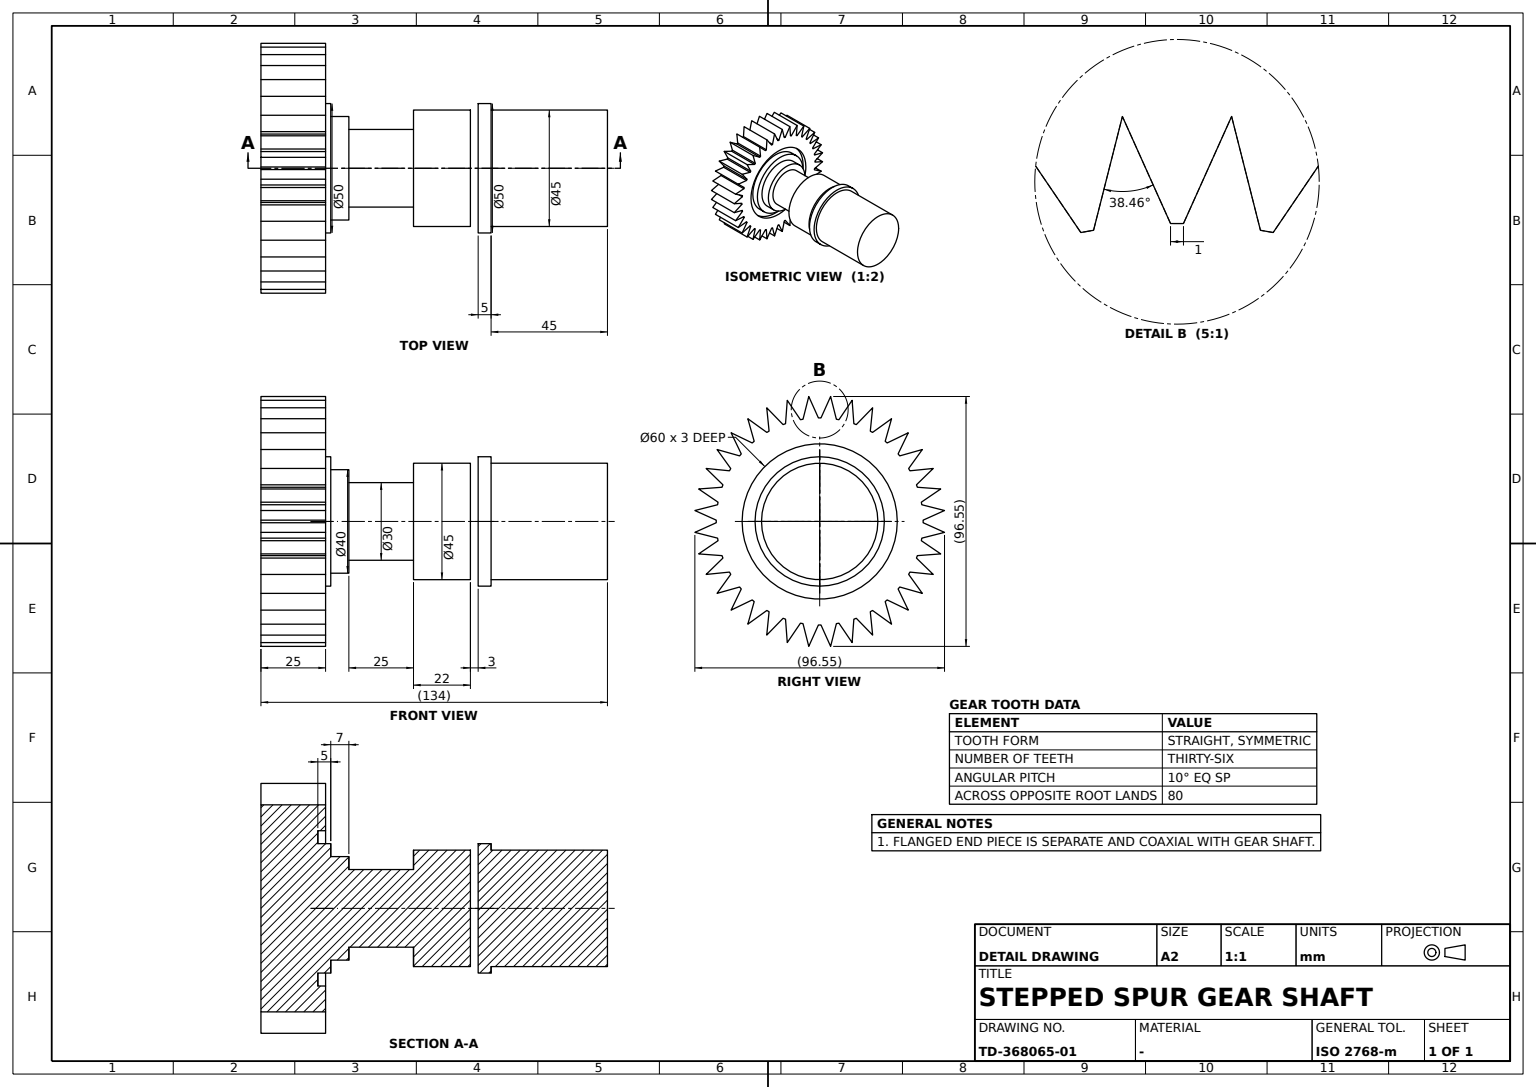
solid
v1 (89,-22.5,0)
v2 (134,-22.5,0)
e1 v1 v2 LINE
v3 (89,22.5,0)
e2 v1 v3 CIRCLE(AX(P(89,0,0),D(1,0,0),D(0,1,0)),22.5)
v4 (134,22.5,0)
e3 v3 v4 LINE
e4 v2 v4 CIRCLE(AX(P(134,0,0),D(1,0,0),D(0,1,0)),22.5)
face CYL(AX(P(71.5,0,0),D(-1,0,0),D(0,1,0)),22.5) [-e1 e2 e3 -e4]
e5 v4 v2 CIRCLE(AX(P(134,0,0),D(1,0,0),D(0,1,0)),22.5)
face PLANE(AX(P(134,0,0),D(1,0,0),D(0,1,0))) [e4 e5]
v5 (84,25,0)
v6 (84,-25,0)
e6 v5 v6 CIRCLE(AX(P(84,0,0),D(1,0,0),D(0,1,0)),25)
v7 (89,-25,0)
e7 v6 v7 LINE
v8 (89,25,0)
e8 v8 v7 CIRCLE(AX(P(89,0,0),D(1,0,0),D(0,1,0)),25)
e9 v5 v8 LINE
face CYL(AX(P(24.5,0,0),D(-1,0,0),D(0,1,0)),25) [e6 e7 -e8 -e9]
e10 v7 v8 CIRCLE(AX(P(89,0,0),D(1,0,0),D(0,1,0)),25)
e11 v3 v1 CIRCLE(AX(P(89,0,0),D(1,0,0),D(0,1,0)),22.5)
face PLANE(AX(P(89,0,0),D(1,0,0),D(0,1,0))) [e10 e8] [-e2 -e11]
face CYL(AX(P(71.5,0,0),D(-1,0,0),D(0,1,0)),22.5) [-e5 -e3 e11 e1]
e12 v6 v5 CIRCLE(AX(P(84,0,0),D(1,0,0),D(0,1,0)),25)
face PLANE(AX(P(84,0,0),D(1,0,0),D(0,1,0))) rev [-e12 -e6]
face CYL(AX(P(24.5,0,0),D(-1,0,0),D(0,1,0)),25) [e9 -e10 -e7 e12]
solid
v9 (0,-39.695086,27.794799)
v10 (25,-39.695086,27.794799)
e13 v9 v10 LINE
v11 (25,-30.963172,25.328482)
e14 v10 v11 LINE
v12 (0,-30.963172,25.328482)
e15 v11 v12 LINE
e16 v9 v12 LINE
face PLANE(AX(P(25,-30.963172,25.328482),D(0,-0.271814264,-0.962349732),D(0,-0.962349732,0.271814264))) rev [e13 e14 e15 -e16]
v13 (25,34.391016,-20.433013)
v14 (0,34.391016,-20.433013)
e17 v13 v14 LINE
v15 (25,39.695086,-27.794799)
e18 v13 v15 LINE
v16 (0,39.695086,-27.794799)
e19 v16 v15 LINE
e20 v14 v16 LINE
face PLANE(AX(P(25,34.391016,-20.433013),D(0,0.811346988,0.584564851),D(0,0.584564851,-0.811346988))) [-e17 e18 -e19 -e20]
v17 (25,-27.794799,-39.695086)
v18 (25,-25.328482,-30.963172)
e21 v17 v18 LINE
v19 (0,-25.328482,-30.963172)
e22 v18 v19 LINE
v20 (0,-27.794799,-39.695086)
e23 v20 v19 LINE
e24 v20 v17 LINE
face PLANE(AX(P(25,-25.328482,-30.963172),D(0,0.962349732,-0.271814264),D(0,-0.271814264,-0.962349732))) rev [e21 e22 -e23 e24]
v21 (0,-20.433013,-34.391016)
e25 v21 v20 LINE
v22 (25,-20.433013,-34.391016)
e26 v22 v21 LINE
e27 v22 v17 LINE
face PLANE(AX(P(25,-20.433013,-34.391016),D(0,0.584564851,-0.811346988),D(0,-0.811346988,-0.584564851))) [-e24 -e25 -e26 e27]
v23 (25,-30.320384,-26.094527)
v24 (0,-30.320384,-26.094527)
e28 v23 v24 LINE
v25 (25,-30.963172,-25.328482)
e29 v23 v25 LINE
v26 (0,-30.963172,-25.328482)
e30 v25 v26 LINE
e31 v24 v26 LINE
face PLANE(AX(P(25,-30.963172,-25.328482),D(0,0.766044443,0.64278761),D(0,0.64278761,-0.766044443))) rev [-e28 e29 e30 -e31]
v27 (27,20,0)
v28 (27,-20,0)
e32 v27 v28 CIRCLE(AX(P(27,0,0),D(1,0,0),D(0,1,0)),20)
e33 v28 v27 CIRCLE(AX(P(27,0,0),D(1,0,0),D(0,1,0)),20)
v29 (27,-25,0)
v30 (27,25,0)
e34 v29 v30 CIRCLE(AX(P(27,0,0),D(1,0,0),D(0,1,0)),25)
e35 v30 v29 CIRCLE(AX(P(27,0,0),D(1,0,0),D(0,1,0)),25)
face PLANE(AX(P(27,0,0),D(1,0,0),D(0,1,0))) [-e32 -e33] [e34 e35]
v31 (0,4.223459,-48.274352)
v32 (25,4.223459,-48.274352)
e36 v31 v32 LINE
v33 (25,0.5,-40)
e37 v32 v33 LINE
v34 (0,0.5,-40)
e38 v33 v34 LINE
e39 v31 v34 LINE
face PLANE(AX(P(25,0.5,-40),D(0,0.911921505,0.410364677),D(0,0.410364677,-0.911921505))) rev [e36 e37 e38 -e39]
v35 (25,-13.210959,37.758715)
v36 (0,-13.210959,37.758715)
e40 v35 v36 LINE
v37 (25,-12.542048,46.807561)
e41 v35 v37 LINE
v38 (0,-12.542048,46.807561)
e42 v38 v37 LINE
e43 v36 v38 LINE
face PLANE(AX(P(25,-13.210959,37.758715),D(0,-0.997278895,0.073721135),D(0,0.073721135,0.997278895))) [-e40 e41 -e42 -e43]
v39 (0,37.758715,-13.210959)
v40 (0,37.416695,-14.150652)
e44 v39 v40 LINE
v41 (25,37.758715,-13.210959)
e45 v41 v39 LINE
v42 (25,37.416695,-14.150652)
e46 v41 v42 LINE
e47 v42 v40 LINE
face PLANE(AX(P(25,37.416695,-14.150652),D(0,-0.939692621,0.342020143),D(0,0.342020143,0.939692621))) rev [-e44 -e45 e46 e47]
v43 (25,20.479554,43.918545)
v44 (25,19.566987,34.891016)
e48 v43 v44 LINE
v45 (0,19.566987,34.891016)
e49 v44 v45 LINE
v46 (0,20.479554,43.918545)
e50 v46 v45 LINE
e51 v46 v43 LINE
face PLANE(AX(P(25,19.566987,34.891016),D(0,-0.994929528,0.100574517),D(0,0.100574517,0.994929528))) rev [e48 e49 -e50 e51]
v47 (25,37.416695,14.150652)
v48 (0,37.416695,14.150652)
e52 v47 v48 LINE
v49 (25,37.758715,13.210959)
e53 v47 v49 LINE
v50 (0,37.758715,13.210959)
e54 v49 v50 LINE
e55 v48 v50 LINE
face PLANE(AX(P(25,37.758715,13.210959),D(0,-0.939692621,-0.342020143),D(0,-0.342020143,0.939692621))) rev [-e52 e53 e54 -e55]
v51 (0,-19.566987,-34.891016)
e56 v51 v21 LINE
v52 (25,-19.566987,-34.891016)
e57 v52 v51 LINE
e58 v52 v22 LINE
face PLANE(AX(P(25,-20.433013,-34.391016),D(0,0.5,0.866025404),D(0,0.866025404,-0.5))) rev [e26 -e56 -e57 e58]
v53 (25,34.891016,19.566987)
v54 (0,34.891016,19.566987)
e59 v53 v54 LINE
v55 (0,34.391016,20.433013)
e60 v55 v54 LINE
v56 (25,34.391016,20.433013)
e61 v56 v55 LINE
e62 v56 v53 LINE
face PLANE(AX(P(25,34.891016,19.566987),D(0,-0.866025404,-0.5),D(0,-0.5,0.866025404))) rev [e59 -e60 -e61 e62]
v57 (0,27.794799,-39.695086)
v58 (25,27.794799,-39.695086)
e63 v57 v58 LINE
v59 (25,20.433013,-34.391016)
e64 v58 v59 LINE
v60 (0,20.433013,-34.391016)
e65 v59 v60 LINE
e66 v57 v60 LINE
face PLANE(AX(P(25,20.433013,-34.391016),D(0,0.584564851,0.811346988),D(0,0.811346988,-0.584564851))) rev [e63 e64 e65 -e66]
v61 (25,-37.416695,14.150652)
v62 (25,-43.918545,20.479554)
e67 v61 v62 LINE
v63 (0,-43.918545,20.479554)
e68 v63 v62 LINE
v64 (0,-37.416695,14.150652)
e69 v64 v63 LINE
e70 v61 v64 LINE
face PLANE(AX(P(25,-37.416695,14.150652),D(0,-0.697512183,-0.716572923),D(0,-0.716572923,0.697512183))) [e67 -e68 -e69 -e70]
v65 (25,-37.758715,13.210959)
e71 v65 v61 LINE
v66 (0,-37.758715,13.210959)
e72 v66 v64 LINE
e73 v65 v66 LINE
face PLANE(AX(P(25,-37.416695,14.150652),D(0,0.939692621,-0.342020143),D(0,-0.342020143,-0.939692621))) rev [e71 e70 -e72 -e73]
v67 (0,-0.5,-40)
e74 v34 v67 LINE
v68 (25,-0.5,-40)
e75 v33 v68 LINE
e76 v68 v67 LINE
face PLANE(AX(P(25,-0.5,-40),D(0,0,1),D(0,1,0))) rev [-e74 -e38 e75 e76]
v69 (25,12.542048,-46.807561)
v70 (25,7.438331,-39.305486)
e77 v69 v70 LINE
v71 (0,7.438331,-39.305486)
e78 v70 v71 LINE
v72 (0,12.542048,-46.807561)
e79 v72 v71 LINE
e80 v72 v69 LINE
face PLANE(AX(P(25,7.438331,-39.305486),D(0,0.82680829,0.562483823),D(0,0.562483823,-0.82680829))) rev [e77 e78 -e79 e80]
v73 (25,40,0.5)
v74 (25,40,-0.5)
e81 v73 v74 LINE
v75 (0,40,-0.5)
e82 v74 v75 LINE
v76 (0,40,0.5)
e83 v76 v75 LINE
e84 v73 v76 LINE
face PLANE(AX(P(25,40,-0.5),D(0,-1,0),D(0,0,1))) rev [e81 e82 -e83 -e84]
v77 (25,30.963172,-25.328482)
e85 v15 v77 LINE
v78 (0,30.963172,-25.328482)
e86 v77 v78 LINE
e87 v16 v78 LINE
face PLANE(AX(P(25,30.963172,-25.328482),D(0,0.271814264,0.962349732),D(0,0.962349732,-0.271814264))) rev [e85 e86 -e87 e19]
v79 (0,-34.265513,-34.265513)
v80 (25,-34.265513,-34.265513)
e88 v79 v80 LINE
v81 (0,-26.094527,-30.320384)
e89 v81 v79 LINE
v82 (25,-26.094527,-30.320384)
e90 v82 v81 LINE
e91 v82 v80 LINE
face PLANE(AX(P(25,-26.094527,-30.320384),D(0,0.434795072,-0.900529425),D(0,-0.900529425,-0.434795072))) [-e88 -e89 -e90 e91]
v83 (0,-46.807561,-12.542048)
v84 (0,-39.305486,-7.438331)
e92 v83 v84 LINE
v85 (25,-46.807561,-12.542048)
e93 v83 v85 LINE
v86 (25,-39.305486,-7.438331)
e94 v85 v86 LINE
e95 v86 v84 LINE
face PLANE(AX(P(25,-39.305486,-7.438331),D(0,0.562483823,-0.82680829),D(0,-0.82680829,-0.562483823))) rev [-e92 e93 e94 e95]
v87 (25,-25.328482,30.963172)
v88 (0,-25.328482,30.963172)
e96 v87 v88 LINE
v89 (25,-27.794799,39.695086)
e97 v87 v89 LINE
v90 (0,-27.794799,39.695086)
e98 v90 v89 LINE
e99 v88 v90 LINE
face PLANE(AX(P(25,-25.328482,30.963172),D(0,-0.962349732,-0.271814264),D(0,-0.271814264,0.962349732))) [-e96 e97 -e98 -e99]
v91 (22,-25,0)
v92 (22,25,0)
e100 v91 v92 CIRCLE(AX(P(22,0,0),D(1,0,0),D(0,1,0)),25)
e101 v92 v91 CIRCLE(AX(P(22,0,0),D(1,0,0),D(0,1,0)),25)
v93 (22,-30,0)
v94 (22,30,0)
e102 v93 v94 CIRCLE(AX(P(22,0,0),D(1,0,0),D(0,1,0)),30)
e103 v94 v93 CIRCLE(AX(P(22,0,0),D(1,0,0),D(0,1,0)),30)
face PLANE(AX(P(22,0,0),D(1,0,0),D(0,1,0))) [-e100 -e101] [e102 e103]
v95 (25,-40,-0.5)
v96 (25,-40,0.5)
e104 v95 v96 LINE
v97 (0,-40,0.5)
e105 v96 v97 LINE
v98 (0,-40,-0.5)
e106 v98 v97 LINE
e107 v95 v98 LINE
face PLANE(AX(P(25,-40,0.5),D(0,1,0),D(0,0,-1))) rev [e104 e105 -e106 -e107]
v99 (0,39.695086,27.794799)
e108 v99 v55 LINE
v100 (25,39.695086,27.794799)
e109 v99 v100 LINE
e110 v100 v56 LINE
face PLANE(AX(P(25,34.391016,20.433013),D(0,-0.811346988,0.584564851),D(0,0.584564851,0.811346988))) rev [e61 -e108 e109 e110]
v101 (25,12.542048,46.807561)
v102 (25,13.210959,37.758715)
e111 v101 v102 LINE
v103 (0,13.210959,37.758715)
e112 v102 v103 LINE
v104 (0,12.542048,46.807561)
e113 v104 v103 LINE
e114 v104 v101 LINE
face PLANE(AX(P(25,13.210959,37.758715),D(0,-0.997278895,-0.073721135),D(0,-0.073721135,0.997278895))) rev [e111 e112 -e113 e114]
v105 (0,19.566987,-34.891016)
v106 (0,20.479554,-43.918545)
e115 v105 v106 LINE
v107 (25,19.566987,-34.891016)
e116 v107 v105 LINE
v108 (25,20.479554,-43.918545)
e117 v107 v108 LINE
e118 v106 v108 LINE
face PLANE(AX(P(25,19.566987,-34.891016),D(0,0.994929528,0.100574517),D(0,0.100574517,-0.994929528))) [-e115 -e116 e117 -e118]
v109 (25,43.918545,-20.479554)
e119 v42 v109 LINE
v110 (0,43.918545,-20.479554)
e120 v110 v109 LINE
e121 v40 v110 LINE
face PLANE(AX(P(25,37.416695,-14.150652),D(0,0.697512183,0.716572923),D(0,0.716572923,-0.697512183))) [e119 -e120 -e121 -e47]
v111 (0,-19.566987,34.891016)
v112 (0,-20.479554,43.918545)
e122 v111 v112 LINE
v113 (25,-19.566987,34.891016)
e123 v113 v111 LINE
v114 (25,-20.479554,43.918545)
e124 v113 v114 LINE
e125 v112 v114 LINE
face PLANE(AX(P(25,-19.566987,34.891016),D(0,-0.994929528,-0.100574517),D(0,-0.100574517,0.994929528))) [-e122 -e123 e124 -e125]
v115 (25,30.320384,-26.094527)
e126 v77 v115 LINE
v116 (0,30.320384,-26.094527)
e127 v115 v116 LINE
e128 v78 v116 LINE
face PLANE(AX(P(25,30.320384,-26.094527),D(0,-0.766044443,0.64278761),D(0,0.64278761,0.766044443))) rev [e126 e127 -e128 -e86]
v117 (0,-20.433013,34.391016)
e129 v117 v111 LINE
v118 (25,-20.433013,34.391016)
e130 v118 v117 LINE
e131 v118 v113 LINE
face PLANE(AX(P(25,-19.566987,34.891016),D(0,0.5,-0.866025404),D(0,-0.866025404,-0.5))) rev [e123 -e129 -e130 e131]
e132 v90 v117 LINE
e133 v89 v118 LINE
face PLANE(AX(P(25,-20.433013,34.391016),D(0,-0.584564851,-0.811346988),D(0,-0.811346988,0.584564851))) rev [-e132 e98 e133 e130]
e134 v91 v29 LINE
e135 v92 v30 LINE
face CYL(AX(P(24.5,0,0),D(-1,0,0),D(0,1,0)),25) [e101 e134 -e35 -e135]
v119 (25,14.150652,-37.416695)
e136 v108 v119 LINE
v120 (0,14.150652,-37.416695)
e137 v119 v120 LINE
e138 v106 v120 LINE
face PLANE(AX(P(25,14.150652,-37.416695),D(0,0.716572923,0.697512183),D(0,0.697512183,-0.716572923))) rev [e136 e137 -e138 e118]
v121 (25,-48.274352,4.223459)
e139 v96 v121 LINE
v122 (0,-48.274352,4.223459)
e140 v122 v121 LINE
e141 v97 v122 LINE
face PLANE(AX(P(25,-40,0.5),D(0,-0.410364677,-0.911921505),D(0,-0.911921505,0.410364677))) [-e105 e139 -e140 -e141]
v123 (25,6.453523,39.479134)
v124 (0,6.453523,39.479134)
e142 v123 v124 LINE
v125 (25,7.438331,39.305486)
e143 v123 v125 LINE
v126 (0,7.438331,39.305486)
e144 v125 v126 LINE
e145 v124 v126 LINE
face PLANE(AX(P(25,7.438331,39.305486),D(0,-0.173648178,-0.984807753),D(0,-0.984807753,0.173648178))) rev [-e142 e143 e144 -e145]
v127 (25,-34.891016,19.566987)
e146 v62 v127 LINE
v128 (0,-34.891016,19.566987)
e147 v127 v128 LINE
e148 v63 v128 LINE
face PLANE(AX(P(25,-34.891016,19.566987),D(0,-0.100574517,-0.994929528),D(0,-0.994929528,0.100574517))) rev [e68 e146 e147 -e148]
v129 (25,20.433013,34.391016)
e149 v44 v129 LINE
v130 (0,20.433013,34.391016)
e150 v129 v130 LINE
e151 v45 v130 LINE
face PLANE(AX(P(25,20.433013,34.391016),D(0,-0.5,-0.866025404),D(0,-0.866025404,0.5))) rev [e149 e150 -e151 -e49]
v131 (25,-14.150652,37.416695)
e152 v131 v35 LINE
v132 (0,-14.150652,37.416695)
e153 v132 v36 LINE
e154 v131 v132 LINE
face PLANE(AX(P(25,-13.210959,37.758715),D(0,0.342020143,-0.939692621),D(0,-0.939692621,-0.342020143))) rev [e152 e40 -e153 -e154]
v133 (25,-7.438331,39.305486)
v134 (25,-6.453523,39.479134)
e155 v133 v134 LINE
v135 (0,-6.453523,39.479134)
e156 v134 v135 LINE
v136 (0,-7.438331,39.305486)
e157 v136 v135 LINE
e158 v133 v136 LINE
face PLANE(AX(P(25,-6.453523,39.479134),D(0,0.173648178,-0.984807753),D(0,-0.984807753,-0.173648178))) rev [e155 e156 -e157 -e158]
v137 (25,-34.391016,20.433013)
e159 v137 v10 LINE
v138 (0,-34.391016,20.433013)
e160 v138 v9 LINE
e161 v137 v138 LINE
face PLANE(AX(P(25,-34.391016,20.433013),D(0,-0.811346988,-0.584564851),D(0,-0.584564851,0.811346988))) [e159 -e13 -e160 -e161]
v139 (25,6.453523,-39.479134)
e162 v139 v32 LINE
v140 (0,6.453523,-39.479134)
e163 v140 v31 LINE
e164 v139 v140 LINE
face PLANE(AX(P(25,6.453523,-39.479134),D(0,0.969326447,-0.245776808),D(0,-0.245776808,-0.969326447))) [e162 -e36 -e163 -e164]
v141 (34,20,0)
v142 (34,-20,0)
e165 v141 v142 CIRCLE(AX(P(34,0,0),D(1,0,0),D(0,1,0)),20)
e166 v142 v141 CIRCLE(AX(P(34,0,0),D(1,0,0),D(0,1,0)),20)
v143 (34,15,0)
v144 (34,-15,0)
e167 v143 v144 CIRCLE(AX(P(34,0,0),D(1,0,0),D(0,1,0)),15)
e168 v144 v143 CIRCLE(AX(P(34,0,0),D(1,0,0),D(0,1,0)),15)
face PLANE(AX(P(34,0,0),D(1,0,0),D(0,1,0))) [e165 e166] [-e167 -e168]
v145 (0,39.305486,7.438331)
v146 (0,39.479134,6.453523)
e169 v145 v146 LINE
v147 (25,39.305486,7.438331)
e170 v147 v145 LINE
v148 (25,39.479134,6.453523)
e171 v147 v148 LINE
e172 v148 v146 LINE
face PLANE(AX(P(25,39.479134,6.453523),D(0,-0.984807753,-0.173648178),D(0,-0.173648178,0.984807753))) rev [-e169 -e170 e171 e172]
v149 (0,-46.807561,12.542048)
v150 (25,-46.807561,12.542048)
e173 v149 v150 LINE
e174 v150 v65 LINE
e175 v149 v66 LINE
face PLANE(AX(P(25,-37.758715,13.210959),D(0,0.073721135,-0.997278895),D(0,-0.997278895,-0.073721135))) rev [e173 e174 e73 -e175]
v151 (0,25.328482,-30.963172)
e176 v151 v57 LINE
v152 (25,25.328482,-30.963172)
e177 v152 v151 LINE
e178 v152 v58 LINE
face PLANE(AX(P(25,25.328482,-30.963172),D(0,0.962349732,0.271814264),D(0,0.271814264,-0.962349732))) [-e63 -e176 -e177 e178]
v153 (25,34.265513,-34.265513)
e179 v115 v153 LINE
v154 (0,34.265513,-34.265513)
e180 v154 v153 LINE
e181 v116 v154 LINE
face PLANE(AX(P(25,30.320384,-26.094527),D(0,0.900529425,0.434795072),D(0,0.434795072,-0.900529425))) [e179 -e180 -e181 -e127]
v155 (25,-37.416695,-14.150652)
v156 (25,-37.758715,-13.210959)
e182 v155 v156 LINE
v157 (0,-37.758715,-13.210959)
e183 v156 v157 LINE
v158 (0,-37.416695,-14.150652)
e184 v158 v157 LINE
e185 v155 v158 LINE
face PLANE(AX(P(25,-37.758715,-13.210959),D(0,0.939692621,0.342020143),D(0,0.342020143,-0.939692621))) rev [e182 e183 -e184 -e185]
v159 (25,-34.391016,-20.433013)
v160 (25,-34.891016,-19.566987)
e186 v159 v160 LINE
v161 (0,-34.891016,-19.566987)
e187 v160 v161 LINE
v162 (0,-34.391016,-20.433013)
e188 v162 v161 LINE
e189 v159 v162 LINE
face PLANE(AX(P(25,-34.891016,-19.566987),D(0,0.866025404,0.5),D(0,0.5,-0.866025404))) rev [e186 e187 -e188 -e189]
v163 (25,39.305486,-7.438331)
v164 (25,46.807561,-12.542048)
e190 v163 v164 LINE
v165 (0,46.807561,-12.542048)
e191 v165 v164 LINE
v166 (0,39.305486,-7.438331)
e192 v166 v165 LINE
e193 v163 v166 LINE
face PLANE(AX(P(25,39.305486,-7.438331),D(0,0.562483823,0.82680829),D(0,0.82680829,-0.562483823))) [e190 -e191 -e192 -e193]
v167 (0,-6.453523,-39.479134)
v168 (0,-7.438331,-39.305486)
e194 v167 v168 LINE
v169 (25,-6.453523,-39.479134)
e195 v169 v167 LINE
v170 (25,-7.438331,-39.305486)
e196 v169 v170 LINE
e197 v170 v168 LINE
face PLANE(AX(P(25,-7.438331,-39.305486),D(0,0.173648178,0.984807753),D(0,0.984807753,-0.173648178))) rev [-e194 -e195 e196 e197]
v171 (25,13.210959,-37.758715)
e198 v119 v171 LINE
v172 (0,13.210959,-37.758715)
e199 v171 v172 LINE
e200 v120 v172 LINE
face PLANE(AX(P(25,13.210959,-37.758715),D(0,-0.342020143,0.939692621),D(0,0.939692621,0.342020143))) rev [-e137 e198 e199 -e200]
v173 (25,48.274352,-4.223459)
e201 v74 v173 LINE
v174 (0,48.274352,-4.223459)
e202 v174 v173 LINE
e203 v75 v174 LINE
face PLANE(AX(P(25,40,-0.5),D(0,0.410364677,0.911921505),D(0,0.911921505,-0.410364677))) [-e82 e201 -e202 -e203]
e204 v171 v69 LINE
e205 v172 v72 LINE
face PLANE(AX(P(25,13.210959,-37.758715),D(0,0.997278895,-0.073721135),D(0,-0.073721135,-0.997278895))) [-e199 e204 -e80 -e205]
v175 (25,-39.479134,6.453523)
v176 (0,-39.479134,6.453523)
e206 v175 v176 LINE
v177 (25,-39.305486,7.438331)
e207 v175 v177 LINE
v178 (0,-39.305486,7.438331)
e208 v177 v178 LINE
e209 v176 v178 LINE
face PLANE(AX(P(25,-39.305486,7.438331),D(0,0.984807753,-0.173648178),D(0,-0.173648178,-0.984807753))) rev [-e206 e207 e208 -e209]
v179 (0,48.274352,4.223459)
e210 v179 v76 LINE
v180 (25,48.274352,4.223459)
e211 v179 v180 LINE
e212 v180 v73 LINE
face PLANE(AX(P(25,40,0.5),D(0,-0.410364677,0.911921505),D(0,0.911921505,0.410364677))) rev [e84 -e210 e211 e212]
v181 (25,26.094527,-30.320384)
v182 (0,26.094527,-30.320384)
e213 v181 v182 LINE
e214 v154 v182 LINE
e215 v153 v181 LINE
face PLANE(AX(P(25,26.094527,-30.320384),D(0,0.434795072,0.900529425),D(0,0.900529425,-0.434795072))) rev [e213 -e214 e180 e215]
v183 (25,25.328482,30.963172)
v184 (25,26.094527,30.320384)
e216 v183 v184 LINE
v185 (0,26.094527,30.320384)
e217 v184 v185 LINE
v186 (0,25.328482,30.963172)
e218 v186 v185 LINE
e219 v183 v186 LINE
face PLANE(AX(P(25,26.094527,30.320384),D(0,-0.64278761,-0.766044443),D(0,-0.766044443,0.64278761))) rev [e216 e217 -e218 -e219]
v187 (0,30.963172,25.328482)
e220 v187 v99 LINE
v188 (25,30.963172,25.328482)
e221 v188 v187 LINE
e222 v188 v100 LINE
face PLANE(AX(P(25,30.963172,25.328482),D(0,-0.271814264,0.962349732),D(0,0.962349732,0.271814264))) [-e220 -e221 e222 -e109]
v189 (25,34.891016,-19.566987)
e223 v109 v189 LINE
v190 (0,34.891016,-19.566987)
e224 v189 v190 LINE
e225 v110 v190 LINE
face PLANE(AX(P(25,34.891016,-19.566987),D(0,0.100574517,0.994929528),D(0,0.994929528,-0.100574517))) rev [e223 e224 -e225 e120]
e226 v79 v24 LINE
e227 v80 v23 LINE
face PLANE(AX(P(25,-30.320384,-26.094527),D(0,0.900529425,-0.434795072),D(0,-0.434795072,-0.900529425))) rev [-e226 e88 e227 e28]
v191 (25,-30.320384,26.094527)
v192 (0,-30.320384,26.094527)
e228 v191 v192 LINE
v193 (25,-34.265513,34.265513)
e229 v191 v193 LINE
v194 (0,-34.265513,34.265513)
e230 v194 v193 LINE
e231 v192 v194 LINE
face PLANE(AX(P(25,-30.320384,26.094527),D(0,-0.900529425,-0.434795072),D(0,-0.434795072,0.900529425))) [-e228 e229 -e230 -e231]
e232 v156 v85 LINE
e233 v157 v83 LINE
face PLANE(AX(P(25,-37.758715,-13.210959),D(0,-0.073721135,-0.997278895),D(0,-0.997278895,0.073721135))) [e232 -e93 -e233 -e183]
v195 (25,43.918545,20.479554)
e234 v195 v47 LINE
v196 (0,43.918545,20.479554)
e235 v196 v48 LINE
e236 v196 v195 LINE
face PLANE(AX(P(25,37.416695,14.150652),D(0,-0.697512183,0.716572923),D(0,0.716572923,0.697512183))) rev [e234 e52 -e235 e236]
v197 (0,34.265513,34.265513)
v198 (0,30.320384,26.094527)
e237 v197 v198 LINE
v199 (25,34.265513,34.265513)
e238 v197 v199 LINE
v200 (25,30.320384,26.094527)
e239 v199 v200 LINE
e240 v200 v198 LINE
face PLANE(AX(P(25,30.320384,26.094527),D(0,-0.900529425,0.434795072),D(0,0.434795072,0.900529425))) rev [-e237 e238 e239 e240]
v201 (0,-4.223459,48.274352)
v202 (0,-0.5,40)
e241 v201 v202 LINE
v203 (25,-4.223459,48.274352)
e242 v201 v203 LINE
v204 (25,-0.5,40)
e243 v203 v204 LINE
e244 v204 v202 LINE
face PLANE(AX(P(25,-0.5,40),D(0,-0.911921505,-0.410364677),D(0,-0.410364677,0.911921505))) rev [-e241 e242 e243 e244]
e245 v165 v39 LINE
e246 v164 v41 LINE
face PLANE(AX(P(25,37.758715,-13.210959),D(0,-0.073721135,0.997278895),D(0,0.997278895,0.073721135))) rev [-e245 e191 e246 e45]
e247 v27 v141 LINE
e248 v28 v142 LINE
face CYL(AX(P(30.5,0,0),D(-1,0,0),D(0,1,0)),20) [e247 -e166 -e248 e33]
v205 (0,4.223459,48.274352)
v206 (25,4.223459,48.274352)
e249 v205 v206 LINE
v207 (0,0.5,40)
e250 v207 v205 LINE
v208 (25,0.5,40)
e251 v208 v207 LINE
e252 v208 v206 LINE
face PLANE(AX(P(25,0.5,40),D(0,-0.911921505,0.410364677),D(0,0.410364677,0.911921505))) [-e249 -e250 -e251 e252]
v209 (0,46.807561,12.542048)
v210 (25,46.807561,12.542048)
e253 v209 v210 LINE
e254 v50 v209 LINE
e255 v49 v210 LINE
face PLANE(AX(P(25,37.758715,13.210959),D(0,0.073721135,0.997278895),D(0,0.997278895,-0.073721135))) [-e253 -e254 -e54 e255]
e256 v12 v192 LINE
e257 v11 v191 LINE
face PLANE(AX(P(25,-30.320384,26.094527),D(0,0.766044443,-0.64278761),D(0,-0.64278761,-0.766044443))) rev [-e256 -e15 e257 e228]
e258 v198 v187 LINE
e259 v200 v188 LINE
face PLANE(AX(P(25,30.963172,25.328482),D(0,-0.766044443,-0.64278761),D(0,-0.64278761,0.766044443))) rev [-e258 -e240 e259 e221]
v211 (59,22.5,0)
v212 (81,22.5,0)
e260 v211 v212 LINE
v213 (81,-22.5,0)
e261 v213 v212 CIRCLE(AX(P(81,0,0),D(1,0,0),D(0,1,0)),22.5)
v214 (59,-22.5,0)
e262 v214 v213 LINE
e263 v214 v211 CIRCLE(AX(P(59,0,0),D(1,0,0),D(0,1,0)),22.5)
face CYL(AX(P(71.5,0,0),D(-1,0,0),D(0,1,0)),22.5) [e260 -e261 -e262 e263]
v215 (25,-30,0)
v216 (25,30,0)
e264 v215 v216 CIRCLE(AX(P(25,0,0),D(1,0,0),D(0,1,0)),30)
e265 v216 v94 LINE
e266 v215 v93 LINE
face CYL(AX(P(23.5,0,0),D(-1,0,0),D(0,1,0)),30) rev [e264 e265 -e102 -e266]
e267 v182 v151 LINE
e268 v181 v152 LINE
face PLANE(AX(P(25,25.328482,-30.963172),D(0,-0.64278761,0.766044443),D(0,0.766044443,0.64278761))) rev [e177 -e267 -e213 e268]
e269 v204 v208 LINE
e270 v202 v207 LINE
face PLANE(AX(P(25,0.5,40),D(0,0,-1),D(0,-1,0))) rev [e269 e251 -e270 -e244]
v217 (0,-39.695086,-27.794799)
v218 (25,-39.695086,-27.794799)
e271 v217 v218 LINE
e272 v218 v159 LINE
e273 v217 v162 LINE
face PLANE(AX(P(25,-34.391016,-20.433013),D(0,0.811346988,-0.584564851),D(0,-0.584564851,-0.811346988))) rev [e271 e272 e189 -e273]
e274 v211 v214 CIRCLE(AX(P(59,0,0),D(1,0,0),D(0,1,0)),22.5)
e275 v212 v213 CIRCLE(AX(P(81,0,0),D(1,0,0),D(0,1,0)),22.5)
face CYL(AX(P(71.5,0,0),D(-1,0,0),D(0,1,0)),22.5) [e274 e262 -e275 -e260]
v219 (59,15,0)
e276 v143 v219 LINE
v220 (59,-15,0)
e277 v220 v219 CIRCLE(AX(P(59,0,0),D(1,0,0),D(0,1,0)),15)
e278 v144 v220 LINE
face CYL(AX(P(46.5,0,0),D(-1,0,0),D(0,1,0)),15) [e276 -e277 -e278 e168]
v221 (0,-26.094527,30.320384)
e279 v221 v88 LINE
v222 (25,-26.094527,30.320384)
e280 v222 v221 LINE
e281 v222 v87 LINE
face PLANE(AX(P(25,-25.328482,30.963172),D(0,0.64278761,-0.766044443),D(0,-0.766044443,-0.64278761))) rev [e96 -e279 -e280 e281]
face PLANE(AX(P(81,0,0),D(1,0,0),D(0,1,0))) [e275 e261]
e282 v219 v220 CIRCLE(AX(P(59,0,0),D(1,0,0),D(0,1,0)),15)
face CYL(AX(P(46.5,0,0),D(-1,0,0),D(0,1,0)),15) [-e282 -e276 e167 e278]
e283 v60 v105 LINE
e284 v71 v140 LINE
v223 (0,-4.223459,-48.274352)
e285 v67 v223 LINE
e286 v223 v167 LINE
v224 (0,-12.542048,-46.807561)
e287 v168 v224 LINE
v225 (0,-13.210959,-37.758715)
e288 v224 v225 LINE
v226 (0,-14.150652,-37.416695)
e289 v225 v226 LINE
v227 (0,-20.479554,-43.918545)
e290 v226 v227 LINE
e291 v227 v51 LINE
e292 v19 v81 LINE
e293 v26 v217 LINE
v228 (0,-43.918545,-20.479554)
e294 v161 v228 LINE
e295 v228 v158 LINE
v229 (0,-39.479134,-6.453523)
e296 v84 v229 LINE
v230 (0,-48.274352,-4.223459)
e297 v229 v230 LINE
e298 v230 v98 LINE
e299 v122 v176 LINE
e300 v178 v149 LINE
e301 v128 v138 LINE
e302 v194 v221 LINE
e303 v112 v132 LINE
e304 v38 v136 LINE
e305 v135 v201 LINE
e306 v205 v124 LINE
e307 v126 v104 LINE
v231 (0,14.150652,37.416695)
e308 v103 v231 LINE
e309 v231 v46 LINE
v232 (0,27.794799,39.695086)
e310 v130 v232 LINE
e311 v232 v186 LINE
e312 v185 v197 LINE
e313 v54 v196 LINE
e314 v209 v145 LINE
e315 v146 v179 LINE
v233 (0,39.479134,-6.453523)
e316 v174 v233 LINE
e317 v233 v166 LINE
e318 v190 v14 LINE
face PLANE(AX(P(0,0,0),D(1,0,0),D(0,1,0))) rev [e87 e128 e181 e214 e267 e176 e66 e283 e115 e138 e200 e205 e79 e284 e163 e39 e74 e285 e286 e194 e287 e288 e289 e290 e291 e56 e25 e23 e292 e89 e226 e31 e293 e273 e188 e294 e295 e184 e233 e92 e296 e297 e298 e106 e141 e299 e209 e300 e175 e72 e69 e148 e301 e160 e16 e256 e231 e302 e279 e99 e132 e129 e122 e303 e153 e43 e304 e157 e305 e241 e270 e250 e306 e145 e307 e113 e308 e309 e50 e151 e310 e311 e218 e312 e237 e258 e220 e108 e60 e313 e235 e55 e254 e314 e169 e315 e210 e83 e203 e316 e317 e192 e245 e44 e121 e225 e318 e20]
e319 v127 v137 LINE
face PLANE(AX(P(25,-34.391016,20.433013),D(0,0.866025404,-0.5),D(0,-0.5,-0.866025404))) rev [-e301 -e147 e319 e161]
v234 (25,39.479134,-6.453523)
e320 v234 v233 LINE
e321 v234 v163 LINE
face PLANE(AX(P(25,39.305486,-7.438331),D(0,-0.984807753,0.173648178),D(0,0.173648178,0.984807753))) rev [e193 -e317 -e320 e321]
e322 v125 v101 LINE
face PLANE(AX(P(25,7.438331,39.305486),D(0,-0.82680829,0.562483823),D(0,0.562483823,0.82680829))) [-e307 -e144 e322 -e114]
v235 (25,-12.542048,-46.807561)
v236 (25,-13.210959,-37.758715)
e323 v235 v236 LINE
e324 v236 v225 LINE
e325 v224 v235 LINE
face PLANE(AX(P(25,-13.210959,-37.758715),D(0,0.997278895,0.073721135),D(0,0.073721135,-0.997278895))) rev [e323 e324 -e288 e325]
e326 v210 v147 LINE
face PLANE(AX(P(25,39.305486,7.438331),D(0,-0.562483823,0.82680829),D(0,0.82680829,0.562483823))) rev [-e314 e253 e326 e170]
v237 (25,14.150652,37.416695)
e327 v237 v231 LINE
e328 v102 v237 LINE
face PLANE(AX(P(25,14.150652,37.416695),D(0,-0.342020143,-0.939692621),D(0,-0.939692621,0.342020143))) rev [e327 -e308 -e112 e328]
e329 v25 v218 LINE
face PLANE(AX(P(25,-30.963172,-25.328482),D(0,0.271814264,-0.962349732),D(0,-0.962349732,-0.271814264))) [-e293 -e30 e329 -e271]
e330 v59 v107 LINE
face PLANE(AX(P(25,19.566987,-34.891016),D(0,-0.5,0.866025404),D(0,0.866025404,0.5))) rev [-e65 e330 e116 -e283]
v238 (25,-43.918545,-20.479554)
e331 v228 v238 LINE
e332 v160 v238 LINE
face PLANE(AX(P(25,-34.891016,-19.566987),D(0,0.100574517,-0.994929528),D(0,-0.994929528,-0.100574517))) [-e331 -e294 -e187 e332]
e333 v134 v203 LINE
face PLANE(AX(P(25,-6.453523,39.479134),D(0,-0.969326447,0.245776808),D(0,0.245776808,0.969326447))) [e333 -e242 -e305 -e156]
e334 v173 v234 LINE
face PLANE(AX(P(25,39.479134,-6.453523),D(0,-0.245776808,0.969326447),D(0,0.969326447,0.245776808))) rev [e202 e334 e320 -e316]
v239 (25,-39.479134,-6.453523)
e335 v239 v229 LINE
v240 (25,-48.274352,-4.223459)
e336 v239 v240 LINE
e337 v230 v240 LINE
face PLANE(AX(P(25,-39.479134,-6.453523),D(0,-0.245776808,-0.969326447),D(0,-0.969326447,0.245776808))) [-e297 -e335 e336 -e337]
v241 (25,-14.150652,-37.416695)
e338 v236 v241 LINE
e339 v241 v226 LINE
face PLANE(AX(P(25,-14.150652,-37.416695),D(0,0.342020143,0.939692621),D(0,0.939692621,-0.342020143))) rev [-e289 -e324 e338 e339]
e340 v86 v239 LINE
face PLANE(AX(P(25,-39.479134,-6.453523),D(0,0.984807753,0.173648178),D(0,0.173648178,-0.984807753))) rev [e335 -e296 -e95 e340]
e341 v177 v150 LINE
face PLANE(AX(P(25,-39.305486,7.438331),D(0,-0.562483823,-0.82680829),D(0,-0.82680829,0.562483823))) [e341 -e173 -e300 -e208]
e342 v189 v13 LINE
face PLANE(AX(P(25,34.391016,-20.433013),D(0,-0.866025404,0.5),D(0,0.5,0.866025404))) rev [-e318 -e224 e342 e17]
e343 v70 v139 LINE
face PLANE(AX(P(25,6.453523,-39.479134),D(0,-0.173648178,0.984807753),D(0,0.984807753,0.173648178))) rev [e164 -e284 -e78 e343]
face PLANE(AX(P(59,0,0),D(1,0,0),D(0,1,0))) rev [e282 e277] [-e263 -e274]
e344 v148 v180 LINE
e345 v53 v195 LINE
e346 v184 v199 LINE
v242 (25,27.794799,39.695086)
e347 v242 v183 LINE
e348 v129 v242 LINE
e349 v237 v43 LINE
e350 v206 v123 LINE
e351 v37 v133 LINE
e352 v114 v131 LINE
e353 v193 v222 LINE
e354 v121 v175 LINE
e355 v240 v95 LINE
e356 v238 v155 LINE
e357 v18 v82 LINE
v243 (25,-20.479554,-43.918545)
e358 v243 v52 LINE
e359 v241 v243 LINE
e360 v170 v235 LINE
v244 (25,-4.223459,-48.274352)
e361 v244 v169 LINE
e362 v68 v244 LINE
e363 v216 v215 CIRCLE(AX(P(25,0,0),D(1,0,0),D(0,1,0)),30)
face PLANE(AX(P(25,0,0),D(1,0,0),D(0,1,0))) [-e190 -e321 -e334 -e201 -e81 -e212 -e344 -e171 -e326 -e255 -e53 -e234 -e345 -e62 -e110 -e222 -e259 -e239 -e346 -e216 -e347 -e348 -e149 -e48 -e349 -e328 -e111 -e322 -e143 -e350 -e252 -e269 -e243 -e333 -e155 -e351 -e41 -e152 -e352 -e124 -e131 -e133 -e97 -e281 -e353 -e229 -e257 -e14 -e159 -e319 -e146 -e67 -e71 -e174 -e341 -e207 -e354 -e139 -e104 -e355 -e336 -e340 -e94 -e232 -e182 -e356 -e332 -e186 -e272 -e329 -e29 -e227 -e91 -e357 -e21 -e27 -e58 -e358 -e359 -e338 -e323 -e360 -e196 -e361 -e362 -e75 -e37 -e162 -e343 -e77 -e204 -e198 -e136 -e117 -e330 -e64 -e178 -e268 -e215 -e179 -e126 -e85 -e18 -e342 -e223 -e119 -e46 -e246] [-e264 -e363]
face PLANE(AX(P(25,-7.438331,-39.305486),D(0,0.82680829,-0.562483823),D(0,-0.562483823,-0.82680829))) [-e325 -e287 -e197 e360]
face CYL(AX(P(30.5,0,0),D(-1,0,0),D(0,1,0)),20) [-e165 -e247 e32 e248]
face PLANE(AX(P(25,-40,-0.5),D(0,0.410364677,-0.911921505),D(0,-0.911921505,-0.410364677))) rev [e107 -e298 e337 e355]
face PLANE(AX(P(25,6.453523,39.479134),D(0,-0.969326447,-0.245776808),D(0,-0.245776808,0.969326447))) rev [e350 e142 -e306 e249]
e364 v223 v244 LINE
face PLANE(AX(P(25,-0.5,-40),D(0,0.911921505,-0.410364677),D(0,-0.410364677,-0.911921505))) [-e76 e362 -e364 -e285]
face PLANE(AX(P(25,-39.479134,6.453523),D(0,0.245776808,-0.969326447),D(0,-0.969326447,-0.245776808))) rev [e206 -e299 e140 e354]
face CYL(AX(P(24.5,0,0),D(-1,0,0),D(0,1,0)),25) [-e134 e100 e135 -e34]
e365 v232 v242 LINE
face PLANE(AX(P(25,25.328482,30.963172),D(0,-0.962349732,0.271814264),D(0,0.271814264,0.962349732))) rev [e219 -e311 e365 e347]
face PLANE(AX(P(25,-26.094527,30.320384),D(0,-0.434795072,-0.900529425),D(0,-0.900529425,0.434795072))) rev [e230 e353 e280 -e302]
face PLANE(AX(P(25,-26.094527,-30.320384),D(0,0.64278761,0.766044443),D(0,0.766044443,-0.64278761))) rev [e357 e90 -e292 -e22]
e366 v227 v243 LINE
face PLANE(AX(P(25,-14.150652,-37.416695),D(0,0.716572923,-0.697512183),D(0,-0.697512183,-0.716572923))) [-e290 -e339 e359 -e366]
face PLANE(AX(P(25,26.094527,30.320384),D(0,-0.434795072,0.900529425),D(0,0.900529425,0.434795072))) [-e312 -e217 e346 -e238]
face PLANE(AX(P(25,39.479134,6.453523),D(0,0.245776808,0.969326447),D(0,0.969326447,-0.245776808))) [e344 -e211 -e315 -e172]
face PLANE(AX(P(25,-14.150652,37.416695),D(0,-0.716572923,-0.697512183),D(0,-0.697512183,0.716572923))) rev [e125 e352 e154 -e303]
face PLANE(AX(P(25,14.150652,37.416695),D(0,-0.716572923,0.697512183),D(0,0.697512183,0.716572923))) [-e327 e349 -e51 -e309]
face PLANE(AX(P(25,-19.566987,-34.891016),D(0,0.994929528,-0.100574517),D(0,-0.100574517,-0.994929528))) rev [e57 -e291 e366 e358]
face PLANE(AX(P(25,20.433013,34.391016),D(0,-0.584564851,0.811346988),D(0,0.811346988,0.584564851))) [-e365 -e310 -e150 e348]
face PLANE(AX(P(25,34.891016,19.566987),D(0,-0.100574517,0.994929528),D(0,0.994929528,0.100574517))) [-e313 -e59 e345 -e236]
face PLANE(AX(P(25,-7.438331,39.305486),D(0,-0.82680829,-0.562483823),D(0,-0.562483823,0.82680829))) rev [e351 e158 -e304 e42]
face PLANE(AX(P(25,-37.416695,-14.150652),D(0,0.697512183,-0.716572923),D(0,-0.716572923,-0.697512183))) rev [-e295 e331 e356 e185]
face PLANE(AX(P(25,-6.453523,-39.479134),D(0,0.969326447,0.245776808),D(0,0.245776808,-0.969326447))) rev [e361 e195 -e286 e364]
face CYL(AX(P(23.5,0,0),D(-1,0,0),D(0,1,0)),30) rev [-e103 -e265 e363 e266]
